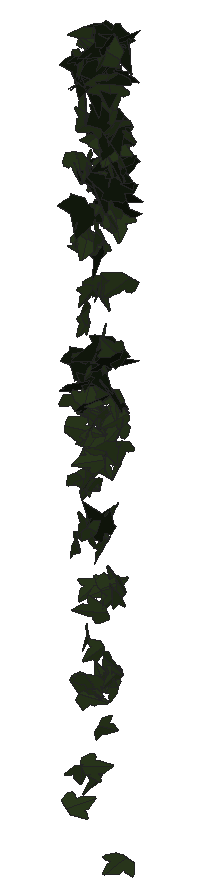
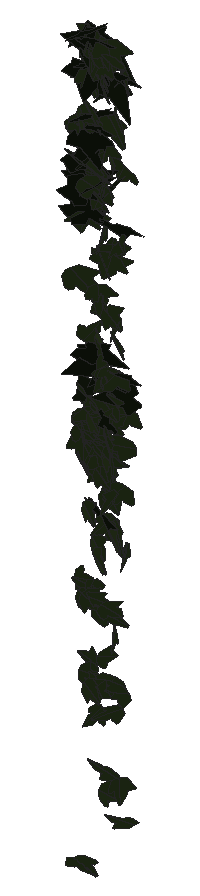
# SketchUp Ruby script. Lengths in inches.
U = 1.inch
M = Sketchup.active_model
def pt(a) = Geom::Point3d.new(a.map { |v| v * U })
def face(e, loops, mat)
  f = e.add_face(loops[0].map { |a| pt(a) })
  loops[1..].each { |l| e.add_face(l.map { |a| pt(a) }).erase! }
  f.material = f.back_material = mat if mat
  f
end
# faces: each face lists its corners as indices into pts; further lists are holes
def faces(e, pts, list, mat = nil) = list.each { |f| face(e, (f[0].is_a?(Array) ? f : [f]).map { |l| l.map { |i| pts[i] } }, mat) }
# xy, xz, yz: faces in a plane at the given z, y or x. An outline is a flat list of corners, or four numbers for a rectangle; further outlines are holes
def ring(l) = l.size == 4 ? [[l[0], l[1]], [l[2], l[1]], [l[2], l[3]], [l[0], l[3]]] : l.each_slice(2).to_a
def flat(e, list, mat, &to3) = list.each { |f| face(e, (f[0].is_a?(Array) ? f : [f]).map { |l| ring(l).map { |u, v| to3.(u, v) } }, mat) }
def xy(e, z, list, mat = nil) = flat(e, list, mat) { |x, y| [x, y, z] }
def xz(e, y, list, mat = nil) = flat(e, list, mat) { |x, z| [x, y, z] }
def yz(e, x, list, mat = nil) = flat(e, list, mat) { |y, z| [x, y, z] }
def lines(e, pts, list) = list.each { |a, b| e.add_line(pt(pts[a]), pt(pts[b])) }
# prism: a flat outline (further loops are holes) pulled along v
def prism(e, loops, v, mat = nil)
  f = face(e, loops, mat); d = Geom::Vector3d.new(v.map { |x| x * U })
  f.pushpull(f.normal.samedirection?(d) ? d.length : -d.length)
end
def box(e, o, s, mat = nil) = prism(e, [[o, [o[0] + s[0], o[1], o[2]], [o[0] + s[0], o[1] + s[1], o[2]], [o[0], o[1] + s[1], o[2]]]], [0, 0, s[2]], mat)
def at(x, y, z, deg = 0) = Geom::Transformation.translation(pt([x, y, z])) * Geom::Transformation.rotation(ORIGIN, Z_AXIS, deg.degrees)
def axes(o, x, y, z) = Geom::Transformation.new([*x, 0, *y, 0, *z, 0, *pt(o).to_a, 1])
def part(name) = M.definitions.add(name)
# library, detail: a bought-in or finely detailed component or shape, given as its bounding box
def library(name, o, s) = part(name).tap { |d| box(d.entities, o, s) }
def detail(e, o, s) = box(e.add_group.entities, o, s)
def put(e, d, t, mat = nil) = e.add_instance(d, t).tap { |i| i.material = mat if mat }
def group(e, t, mat = nil) = e.add_group.tap { |g| g.transformation = t; g.material = mat if mat }.entities
root = M.entities
M.materials.add("1026 AP 7946 SUNNY SIDE UP").color = [254, 231, 186]
M.materials.add("efeu1").color = [18, 25, 13]
M.materials.add("efeu2").color = [43, 57, 29]
c1 = part("ivyleaf_10")
p = [[0,0.5,-0.03],[-0.0625,2.02,-0.43],[-0.19,2.01,-0.46],[-0.54,1.05,-0.29],[-0.52,0.625,-0.18],[-0.83,0.76,-0.28],
  [-1.16,0.64,-0.33],[-1.15,0.33,-0.24],[-0.77,-0.39,0.02],[-0.3,-0.51,0.16],[0.04,-0.48,0.23],[-0.02,2.01,-0.4375],
  [-0.06,2.01,-0.43],[0.04,-0.49,0.23],[0.67,-0.49,0.14],[1.38,0.36,-0.2],[1.375,0.51,-0.24],[0.81,0.65,-0.19],
  [0.62,0.59,-0.15],[0.6,1.09,-0.28],[0.5,1.23,-0.31]]
faces(c1.entities,p,[[0,1,2,3,4,5,6,7,8,9,10],[11,12,0,13,14,15,16,17,18,19,20]],"efeu2")
c2 = part("ivyleaf_9")
p = [[1.54,2.16,1.25],[1.36,2.04,1.19],[-0.21,0.99,0.68],[-0.71,1.11,0.82],[-0.85,0.86,0.67],[-0.8,0.17,0.21],
  [-0.9,-0.01,0.1],[-0.67,-0.16,-0.02],[-0.08,-0.08,-0.05],[-0.03,-0.6,-0.4],[0.65,-0.88,-0.66],[0.83,-0.6,-0.49],
  [1.29,-0.42,-0.43],[1.8125,-0.07,-0.26],[1.21,0.44,0.15]]
faces(c2.entities,p,[[0,1,2,3,4,5,6,7,8,9,10,11,12,13,14]],"efeu1")
put(root,c1,axes([98.51,212.3,259.13],[-0.27937,-0.11894,-0.10126],[0.16168,0.02502,-0.21427],[0.19891,-0.18739,0.03195]),"1026 AP 7946 SUNNY SIDE UP")
put(root,c1,axes([98.56,212.43,263.14],[0.0391,0.17474,-0.14079],[-0.04815,-0.13104,-0.19029],[-0.37047,0.03547,0.00987]),"1026 AP 7946 SUNNY SIDE UP")
put(root,c1,axes([98.64,212.66,261.58],[-0.05241,-0.19052,0.11214],[-0.0155,-0.10979,-0.19972],[0.34552,-0.03382,0.00805]),"1026 AP 7946 SUNNY SIDE UP")
put(root,c1,axes([98.7,212.33,261.15],[-0.02487,0.03429,0.22922],[-0.17054,0.1886,-0.03714],[-0.32536,-0.10148,0.00194]),"1026 AP 7946 SUNNY SIDE UP")
put(root,c1,axes([98.63,212.31,250.48],[-0.13312,-0.18944,-0.0198],[0.02536,0.01265,-0.21346],[0.29817,-0.08566,0.00931]),"1026 AP 7946 SUNNY SIDE UP")
put(root,c1,axes([98.66,212.21,267.14],[0.21762,-0.19818,-0.09251],[-0.05141,0.08493,-0.24763],[0.3375,0.14073,0.02193]),"1026 AP 7946 SUNNY SIDE UP")
put(root,c1,axes([98.61,212.11,255.87],[0.08491,-0.17723,-0.12547],[0.04251,0.12919,-0.18207],[0.33455,0.02856,0.05498]),"1026 AP 7946 SUNNY SIDE UP")
put(root,c1,axes([98.64,212.44,260.89],[0.20499,-0.14401,-0.02204],[-0.03094,0.00911,-0.2009],[0.24458,0.12186,-0.00694]),"1026 AP 7946 SUNNY SIDE UP")
put(root,c2,axes([98.64,212.48,263.58],[-0.31071,-0.12436,-0.07465],[0.13892,-0.00184,-0.23189],[0.19656,-0.19529,0.04589]),"1026 AP 7946 SUNNY SIDE UP")
put(root,c2,axes([98.81,212.31,266.75],[-0.07178,0.25204,-0.03444],[0.00058,-0.03588,-0.27404],[-0.43207,-0.04192,0.00535]),"1026 AP 7946 SUNNY SIDE UP")
put(root,c1,axes([98.47,212.21,249.57],[0.1939,-0.0085,-0.16852],[0.22459,0.10571,0.10591],[0.12594,-0.17543,0.07058]),"1026 AP 7946 SUNNY SIDE UP")
put(root,c1,axes([98.69,212.43,258.09],[0.0331,-0.17595,-0.11475],[-0.0054,0.11064,-0.18171],[0.32656,0.01966,0.00863]),"1026 AP 7946 SUNNY SIDE UP")
put(root,c1,axes([98.75,212.6,254.67],[-0.13776,-0.09753,0.15854],[-0.03053,-0.16535,-0.11989],[0.2856,-0.06472,0.06366]),"1026 AP 7946 SUNNY SIDE UP")
put(root,c2,axes([98.49,212.11,259.4375],[0.25239,0.03969,0.18222],[0.21659,0.12714,-0.14975],[-0.20151,0.18637,0.06728]),"1026 AP 7946 SUNNY SIDE UP")
put(root,c1,axes([98.76,212.52,267.7],[-0.25265,-0.20537,0.01811],[0.0007,-0.02446,-0.27142],[0.35021,-0.14811,0.01361]),"1026 AP 7946 SUNNY SIDE UP")
put(root,c1,axes([98.42,212.33,258.4],[-0.01641,-0.02412,-0.23445],[0.37076,0.02531,-0.01297],[0.04498,-0.21743,0.02139]),"1026 AP 7946 SUNNY SIDE UP")
put(root,c1,axes([98.6,212.31,257.33],[-0.20644,-0.11253,-0.14995],[0.18656,0.08385,-0.17732],[0.22005,-0.17665,0.00967]),"1026 AP 7946 SUNNY SIDE UP")
put(root,c1,axes([98.7,212.56,262.8],[-0.3743,-0.00639,-0.02967],[0.04805,-0.03659,-0.2333],[0.00288,-0.21918,0.03667]),"1026 AP 7946 SUNNY SIDE UP")
put(root,c1,axes([98.91,212.42,258.85],[-0.2398,0.00932,-0.15753],[-0.24756,0.02224,0.15158],[0.03815,0.20285,-0.00651]),"1026 AP 7946 SUNNY SIDE UP")
put(root,c1,axes([98.72,212.42,256.24],[0.1317,-0.18099,0.0391],[0.01121,-0.0396,-0.20543],[0.2909,0.08347,-0.00979]),"1026 AP 7946 SUNNY SIDE UP")
put(root,c1,axes([98.93,212.24,265.76],[-0.29804,0.04713,0.15883],[-0.25334,0.0093,-0.19292],[-0.07154,-0.22927,0.02148]),"1026 AP 7946 SUNNY SIDE UP")
put(root,c1,axes([98.71,212.42,257.18],[-0.01521,0.1355,0.17254],[-0.0448,0.15754,-0.14275],[-0.3523,-0.02588,0.01071]),"1026 AP 7946 SUNNY SIDE UP")
put(root,c2,axes([98.67,212.45,260.06],[-0.25441,-0.13473,-0.09736],[0.13066,0.04743,-0.2145],[0.24116,-0.16783,0.01351]),"1026 AP 7946 SUNNY SIDE UP")
put(root,c1,axes([98.56,212.23,264.79],[0.31903,-0.04945,0.11744],[0.17921,-0.03232,-0.20846],[0.10007,0.21553,-0.00108]),"1026 AP 7946 SUNNY SIDE UP")
put(root,c1,axes([98.92,212.13,256.26],[-0.23981,0.10446,0.18077],[-0.25733,0.06726,-0.18802],[-0.19073,-0.22208,0.02638]),"1026 AP 7946 SUNNY SIDE UP")
put(root,c1,axes([98.81,212.42,262.64],[-0.3139,-0.13165,-0.04887],[-0.07982,-0.0075,0.24533],[-0.20463,0.20488,-0.02072]),"1026 AP 7946 SUNNY SIDE UP")
put(root,c1,axes([98.64,212.48,260.07],[-0.27784,-0.10961,-0.13621],[0.19397,0.04971,-0.213],[0.18681,-0.21463,0.01858]),"1026 AP 7946 SUNNY SIDE UP")
put(root,c1,axes([98.83,212.42,257.21],[-0.11923,-0.19489,0.07201],[-0.02811,-0.06918,-0.21568],[0.32494,-0.07749,0.00777]),"1026 AP 7946 SUNNY SIDE UP")
put(root,c1,axes([98.75,212.36,262.96],[0.24998,0.15657,-0.06162],[-0.04989,-0.05398,-0.2303],[-0.27997,0.14941,-0.01399]),"1026 AP 7946 SUNNY SIDE UP")
put(root,c1,axes([98.75,212.61,258.21],[0.0492,-0.16845,0.14669],[0.07592,-0.13609,-0.17639],[0.33941,0.05486,0.01819]),"1026 AP 7946 SUNNY SIDE UP")
put(root,c2,axes([98.96,212.17,267.46],[-0.18866,0.20878,-0.03742],[0.00466,-0.04111,-0.25315],[-0.3601,-0.10991,0.01633]),"1026 AP 7946 SUNNY SIDE UP")
put(root,c1,axes([98.6,212.42,266.15],[0.16854,-0.13767,0.21387],[0.24806,-0.13848,-0.17866],[0.30445,0.18904,0.02717]),"1026 AP 7946 SUNNY SIDE UP")
put(root,c1,axes([98.83,212.49,258.63],[0.07149,-0.19155,-0.08157],[-0.04031,0.07412,-0.20225],[0.32276,0.05169,-0.00719]),"1026 AP 7946 SUNNY SIDE UP")
put(root,c1,axes([98.95,212.46,259.375],[-0.26546,-0.0683,0.11549],[-0.15441,-0.06207,-0.18262],[0.15391,-0.18008,0.01597]),"1026 AP 7946 SUNNY SIDE UP")
put(root,c1,axes([98.87,212.55,258.04],[-0.2726,-0.1235,0.03485],[-0.03129,-0.03195,-0.21681],[0.21525,-0.16104,0.01263]),"1026 AP 7946 SUNNY SIDE UP")
put(root,c2,axes([98.79,212.36,267.02],[-0.32616,-0.1046,-0.10236],[0.18194,-0.00527,-0.22775],[0.15498,-0.21394,0.05195]),"1026 AP 7946 SUNNY SIDE UP")
put(root,c2,axes([98.65,212.44,264.46],[0.14434,-0.22674,-0.01818],[-0.01554,0.01365,-0.25189],[0.35712,0.09224,-0.00361]),"1026 AP 7946 SUNNY SIDE UP")
put(root,c1,axes([98.68,212.36,252.18],[-0.03252,-0.09944,-0.18967],[0.23523,0.12159,-0.08452],[0.22895,-0.13905,0.05989]),"1026 AP 7946 SUNNY SIDE UP")
put(root,c1,axes([98.79,212.44,257.34],[0.04933,-0.08937,0.20495],[0.08983,-0.19114,-0.09861],[0.33172,0.06505,-0.00378]),"1026 AP 7946 SUNNY SIDE UP")
put(root,c1,axes([98.63,212.25,252.57],[-0.14215,0.00609,-0.19948],[0.29393,-0.05353,-0.09194],[-0.08022,-0.20692,0.01662]),"1026 AP 7946 SUNNY SIDE UP")
put(root,c1,axes([98.79,212.25,259.16],[0.26711,0.08182,-0.04599],[0.05247,0.03555,0.18951],[0.14875,-0.15948,0.01573]),"1026 AP 7946 SUNNY SIDE UP")
put(root,c1,axes([98.88,212.65,257.78],[-0.01609,-0.19014,0.09831],[0.01082,-0.09687,-0.19642],[0.33511,-0.006,0.01106]),"1026 AP 7946 SUNNY SIDE UP")
put(root,c2,axes([98.71,212.31,258.92],[0.14653,0.19149,-0.00182],[-0.02185,0.01039,0.22436],[0.32441,-0.08579,0.01594]),"1026 AP 7946 SUNNY SIDE UP")
put(root,c1,axes([98.82,212.67,261.57],[0.0062,-0.14525,-0.12528],[0.00136,-0.11514,0.15394],[-0.31463,-0.00336,-0.0018]),"1026 AP 7946 SUNNY SIDE UP")
put(root,c1,axes([98.92,212.47,258.3],[0.21092,0.1292,-0.12172],[-0.12844,-0.08725,-0.19305],[-0.26451,0.14539,-0.00332]),"1026 AP 7946 SUNNY SIDE UP")
put(root,c1,axes([98.85,212.51,259.88],[-0.00044,-0.02629,0.21402],[0.09057,-0.19314,-0.02977],[0.33067,0.05287,0.00844]),"1026 AP 7946 SUNNY SIDE UP")
put(root,c1,axes([99.13,212.3125,254.32],[-0.09911,-0.00675,0.21605],[-0.29908,-0.09071,-0.06242],[0.13944,-0.19935,0.01968]),"1026 AP 7946 SUNNY SIDE UP")
put(root,c1,axes([98.9,212.49,250.27],[0.03302,-0.12848,0.16499],[0.02266,-0.1604,-0.13484],[0.32294,0.02439,-0.00741]),"1026 AP 7946 SUNNY SIDE UP")
put(root,c1,axes([99.03,212.33,257.82],[-0.10683,0.00899,0.20822],[-0.1252,-0.19014,-0.01881],[0.30566,-0.07474,0.06507]),"1026 AP 7946 SUNNY SIDE UP")
put(root,c1,axes([98.81,212.34,264.8],[-0.03844,0.04428,-0.23709],[0.06371,-0.21933,-0.05399],[-0.37903,-0.04135,0.01497]),"1026 AP 7946 SUNNY SIDE UP")
put(root,c1,axes([98.85,212.59,267.46],[0.4133,0.0296,-0.00112],[0.0025,-0.02394,-0.26165],[-0.05024,0.24229,-0.02225]),"1026 AP 7946 SUNNY SIDE UP")
put(root,c1,axes([98.95,212.07,253.8],[0.06144,-0.13569,-0.16844],[-0.01402,0.16428,-0.14236],[0.33287,0.03197,0.02509]),"1026 AP 7946 SUNNY SIDE UP")
put(root,c1,axes([98.92,212.65,260.23],[0.01419,0.05061,-0.20662],[-0.05246,-0.19117,-0.05758],[-0.33571,0.03201,0.00027]),"1026 AP 7946 SUNNY SIDE UP")
put(root,c1,axes([98.8125,212.59,266.8],[0.14377,-0.14618,0.19051],[0.17448,-0.14794,-0.18261],[0.35264,0.1328,0.01268]),"1026 AP 7946 SUNNY SIDE UP")
put(root,c1,axes([98.99,212.3,264.31],[-0.1231,0.16229,0.12319],[-0.10423,0.09588,-0.18835],[-0.31906,-0.09394,0.014]),"1026 AP 7946 SUNNY SIDE UP")
put(root,c1,axes([98.97,212.42,258.94],[-0.26949,-0.09574,-0.00046],[0.01282,-0.0141,-0.19793],[0.16202,-0.15813,0.01489]),"1026 AP 7946 SUNNY SIDE UP")
put(root,c1,axes([98.72,212.62,258.68],[0.14584,-0.03881,0.19813],[0.28165,-0.07065,-0.10397],[0.12671,0.2017,0.00307]),"1026 AP 7946 SUNNY SIDE UP")
put(root,c1,axes([98.99,212.55,261.97],[-0.19522,-0.17849,-0.0024],[0.02161,-0.00831,-0.22685],[0.30222,-0.1147,0.01468]),"1026 AP 7946 SUNNY SIDE UP")
put(root,c2,axes([98.78,212.33,259.95],[-0.08489,-0.0751,-0.20496],[0.2101,0.1451,-0.09401],[0.27687,-0.13314,0.0085]),"1026 AP 7946 SUNNY SIDE UP")
put(root,c1,axes([98.93,212.21,252.72],[-0.31487,-0.04415,-0.07122],[0.1122,-0.00511,-0.21034],[0.06296,-0.2117,0.01864]),"1026 AP 7946 SUNNY SIDE UP")
put(root,c1,axes([98.96,212.625,255.76],[0.15168,-0.18378,0.09964],[0.05257,-0.09267,-0.214],[0.32307,0.10136,-0.01196]),"1026 AP 7946 SUNNY SIDE UP")
put(root,c1,axes([98.89,212.6,261.67],[-0.20873,0.08763,-0.10783],[0.10935,-0.08274,-0.1606],[-0.20018,-0.13657,0.02471]),"1026 AP 7946 SUNNY SIDE UP")
put(root,c2,axes([98.82,212.39,266.625],[0.04333,-0.23865,0.0913],[0.01307,-0.08807,-0.25817],[0.43181,0.02662,-0.00135]),"1026 AP 7946 SUNNY SIDE UP")
put(root,c1,axes([99,212.41,253.35],[-0.05101,-0.04646,0.20196],[0.03258,-0.19855,-0.04604],[0.31552,0.01299,0.0374]),"1026 AP 7946 SUNNY SIDE UP")
put(root,c1,axes([98.99,212.5,264.29],[-0.35077,0.08538,-0.0237],[0.02606,-0.02229,-0.24573],[-0.13678,-0.2232,0.01397]),"1026 AP 7946 SUNNY SIDE UP")
put(root,c2,axes([98.95,212.5,262.72],[-0.18407,0.03122,-0.19618],[0.28013,-0.08249,-0.12047],[-0.14672,-0.19667,0.01609]),"1026 AP 7946 SUNNY SIDE UP")
put(root,c1,axes([99,212.5,267.29],[-0.3934,0.08999,-0.04134],[0.04673,-0.03845,-0.26528],[-0.16036,-0.23197,0.02411]),"1026 AP 7946 SUNNY SIDE UP")
put(root,c1,axes([99.15,212.62,254.77],[-0.16653,-0.02914,0.17857],[-0.12282,-0.17366,-0.08019],[0.24787,-0.10563,0.08023]),"1026 AP 7946 SUNNY SIDE UP")
put(root,c1,axes([99.11,212.49,257.97],[-0.11314,-0.17832,0.14224],[-0.06082,-0.1341,-0.19852],[0.35036,-0.08086,0.01147]),"1026 AP 7946 SUNNY SIDE UP")
put(root,c1,axes([99.21,212.61,264.4],[-0.1747,-0.09415,0.19935],[-0.14618,-0.17141,-0.14518],[0.32467,-0.12783,0.0419]),"1026 AP 7946 SUNNY SIDE UP")
put(root,c1,axes([98.9,212.52,259.97],[0.01188,-0.03247,-0.20074],[0.16152,-0.16141,0.03155],[-0.27894,-0.09484,0.00972]),"1026 AP 7946 SUNNY SIDE UP")
put(root,c1,axes([99.09,212.4375,265.28],[-0.39106,-0.06687,-0.01707],[0.03446,-0.01607,-0.25604],[0.11115,-0.2303,0.01932]),"1026 AP 7946 SUNNY SIDE UP")
put(root,c1,axes([99.09,212.35,260.55],[0.14282,-0.13579,0.13688],[-0.09682,0.11684,0.1723],[-0.3036,-0.10113,0.00944]),"1026 AP 7946 SUNNY SIDE UP")
put(root,c1,axes([98.83,212.3,250.59],[0.14585,-0.06022,-0.1841],[0.28577,-0.0232,0.1053],[-0.07717,-0.19969,0.04199]),"1026 AP 7946 SUNNY SIDE UP")
put(root,c1,axes([99.08,212.23,263.22],[0.11176,-0.16866,-0.19047],[0.03383,0.19468,-0.1742],[0.39094,0.03137,0.06953]),"1026 AP 7946 SUNNY SIDE UP")
put(root,c2,axes([99.26,212.54,260.47],[0.00297,-0.01479,-0.25364],[-0.11877,-0.23433,0.01254],[-0.36907,0.07529,-0.00607]),"1026 AP 7946 SUNNY SIDE UP")
put(root,c1,axes([99.02,212.39,257.8],[-0.20222,-0.14229,-0.09098],[0.15478,0.02853,-0.19177],[0.23302,-0.14244,0.04843]),"1026 AP 7946 SUNNY SIDE UP")
put(root,c1,axes([99.18,212.41,252.55],[0.29749,0.01746,0.10047],[-0.15501,0.01435,0.19465],[0.01398,-0.21232,0.02016]),"1026 AP 7946 SUNNY SIDE UP")
put(root,c1,axes([99.35,212.52,264.85],[-0.28601,0.07589,-0.16491],[-0.22965,0.07649,0.19856],[0.18198,0.2158,-0.00862]),"1026 AP 7946 SUNNY SIDE UP")
put(root,c1,axes([99.16,212.55,258.93],[0.0244,-0.20982,0.06757],[0.01133,-0.06642,-0.21712],[0.34604,0.01697,0.00234]),"1026 AP 7946 SUNNY SIDE UP")
put(root,c1,axes([99.13,212.47,264.1],[0.30419,-0.18857,0.02078],[0.00339,-0.02815,-0.27782],[0.29837,0.19257,-0.01803]),"1026 AP 7946 SUNNY SIDE UP")
put(root,c1,axes([98.9,212.65,258.17],[0.05188,-0.04894,-0.23021],[0.2716,-0.14227,0.05761],[-0.23518,-0.1751,0.01575]),"1026 AP 7946 SUNNY SIDE UP")
put(root,c1,axes([99.17,212.66,252.7],[0.00421,-0.19365,0.09972],[0.00482,-0.09786,-0.20008],[0.34116,0.00377,0.0016]),"1026 AP 7946 SUNNY SIDE UP")
put(root,c1,axes([99.25,212.49,263.65],[-0.33224,0.00236,-0.05382],[-0.08442,0.02268,0.20861],[0.01343,0.2008,-0.02009]),"1026 AP 7946 SUNNY SIDE UP")
put(root,c2,axes([99.23,212.53,265.48],[0.17339,0.14884,-0.14041],[-0.10257,-0.11944,-0.19431],[-0.32305,0.11781,-0.01366]),"1026 AP 7946 SUNNY SIDE UP")
put(root,c2,axes([99.39,212.09,256.4],[-0.05623,0.09418,0.24728],[-0.1681,0.21451,-0.10209],[-0.36809,-0.11235,0.00885]),"1026 AP 7946 SUNNY SIDE UP")
put(root,c1,axes([99.1875,212.39,255.95],[0.01516,-0.19879,0.05062],[-0.00178,-0.05038,-0.2053],[0.32242,0.00907,-0.00351]),"1026 AP 7946 SUNNY SIDE UP")
put(root,c2,axes([99.07,212.52,264.36],[-0.04317,-0.23907,0.01891],[-0.00146,-0.01973,-0.24802],[0.37718,-0.02744,0.0012]),"1026 AP 7946 SUNNY SIDE UP")
put(root,c1,axes([99.09,212.0625,256.36],[-0.12191,-0.12486,-0.16671],[0.15397,0.12836,-0.15028],[0.2811,-0.12446,0.01002]),"1026 AP 7946 SUNNY SIDE UP")
put(root,c1,axes([99.19,212.6875,254.8],[-0.05059,-0.16572,0.15327],[0.02261,-0.15248,-0.17159],[0.35044,-0.01409,0.0332]),"1026 AP 7946 SUNNY SIDE UP")
put(root,c2,axes([99.28,212.63,267.72],[-0.37175,-0.09723,0.01009],[-0.00117,-0.02468,-0.25575],[0.16604,-0.21786,0.02078]),"1026 AP 7946 SUNNY SIDE UP")
put(root,c1,axes([98.94,212.48,266.82],[0.14659,-0.09669,0.20939],[0.30651,-0.08873,-0.1327],[0.21131,0.19579,0.04723]),"1026 AP 7946 SUNNY SIDE UP")
put(root,c1,axes([99.125,212.46,267.72],[-0.14475,0.19883,-0.07155],[0.0347,-0.06673,-0.23242],[-0.35582,-0.0874,0.00644]),"1026 AP 7946 SUNNY SIDE UP")
put(root,c1,axes([99.35,212.63,258.81],[0.04839,0.08916,0.22234],[-0.17094,-0.18662,0.09452],[0.32414,-0.11173,0.01666]),"1026 AP 7946 SUNNY SIDE UP")
put(root,c1,axes([99.55,212.2,267.56],[0.07075,0.07181,0.27262],[-0.44743,0.0041,0.04517],[0.01263,-0.25708,0.07301]),"1026 AP 7946 SUNNY SIDE UP")
put(root,c1,axes([99.42,212.32,263.47],[-0.19613,0.08259,-0.15324],[-0.18402,0.09568,0.15298],[0.21384,0.15809,-0.0089]),"1026 AP 7946 SUNNY SIDE UP")
put(root,c1,axes([99.27,212.34,267.43],[-0.00084,-0.19379,-0.15786],[0.01382,0.14484,-0.20534],[0.41055,-0.00527,0.00659]),"1026 AP 7946 SUNNY SIDE UP")
put(root,c1,axes([99.3,212.46,266.08],[0.25064,-0.19225,-0.05334],[-0.06549,0.02996,-0.25877],[0.32965,0.15213,-0.01085]),"1026 AP 7946 SUNNY SIDE UP")
put(root,c1,axes([99.3,212.32,266.87],[-0.20472,-0.22447,-0.00255],[0.02293,-0.00788,-0.27239],[0.38035,-0.12034,0.01505]),"1026 AP 7946 SUNNY SIDE UP")
put(root,c1,axes([99.13,212.47,264.63],[0.26061,-0.10514,0.1217],[0.1574,-0.06819,-0.20013],[0.21266,0.17932,-0.00102]),"1026 AP 7946 SUNNY SIDE UP")
put(root,c1,axes([99.1875,212.41,257.9],[0.01978,-0.07689,-0.17308],[0.04168,-0.15878,0.08104],[-0.29948,-0.02718,-0.00015]),"1026 AP 7946 SUNNY SIDE UP")
put(root,c1,axes([99.26,212.48,264.75],[0.3648,-0.06025,-0.03795],[-0.04196,0.04111,-0.24438],[0.10251,0.23123,0.03504]),"1026 AP 7946 SUNNY SIDE UP")
put(root,c1,axes([99.28,212.48,266.84],[-0.20561,-0.17786,-0.04612],[0.0578,0.02603,-0.22958],[0.30432,-0.12512,0.01244]),"1026 AP 7946 SUNNY SIDE UP")
put(root,c2,axes([99.4,212.41,267.69],[-0.01814,-0.02384,-0.24178],[-0.01211,-0.22563,0.02274],[-0.38478,0.00822,0.01068]),"1026 AP 7946 SUNNY SIDE UP")
put(root,c2,axes([99.57,212.5,264.84],[-0.22791,0.17836,0.08616],[-0.16261,0.02215,-0.23],[-0.2878,-0.15376,0.06173]),"1026 AP 7946 SUNNY SIDE UP")
put(root,c2,axes([99.15,212.33,260.12],[0.19177,0.12467,0.19431],[0.2139,0.12971,-0.17885],[-0.2828,0.18265,-0.00351]),"1026 AP 7946 SUNNY SIDE UP")
put(root,c2,axes([99.29,212.47,266.95],[0.27351,0.12665,-0.08236],[-0.0845,-0.06335,-0.21946],[-0.23849,0.16769,-0.01669]),"1026 AP 7946 SUNNY SIDE UP")
put(root,c1,axes([99.45,212.31,252.69],[0.1287,-0.1055,-0.18228],[-0.19127,0.1281,-0.13638],[0.26041,0.14623,-0.01009]),"1026 AP 7946 SUNNY SIDE UP")
put(root,c2,axes([99.13,212.63,265.08],[0.10328,-0.23495,0.07659],[0.01956,-0.07506,-0.25163],[0.38764,0.06638,-0.00771]),"1026 AP 7946 SUNNY SIDE UP")
put(root,c1,axes([99.38,212.55,254.74],[-0.06566,-0.15869,0.12767],[-0.03589,-0.12294,-0.1696],[0.31544,-0.04702,0.00728]),"1026 AP 7946 SUNNY SIDE UP")
put(root,c2,axes([99.34,212.54,265.64],[-0.32122,-0.1331,-0.05703],[0.09117,0.01289,-0.24658],[0.22448,-0.19569,0.01854]),"1026 AP 7946 SUNNY SIDE UP")
put(root,c2,axes([99.24,212.4,267.04],[-0.17957,-0.21721,-0.06582],[0.07597,0.04319,-0.2571],[0.3743,-0.11298,0.02061]),"1026 AP 7946 SUNNY SIDE UP")
put(root,c2,axes([99.46,212.65,264.97],[0.00581,0.03068,-0.22619],[-0.05785,-0.20892,-0.03592],[-0.35845,0.03421,0.00213]),"1026 AP 7946 SUNNY SIDE UP")
put(root,c1,axes([99.35,212.49,256.74],[0.04266,-0.19718,0.04041],[0.00153,-0.04058,-0.20523],[0.31646,0.02677,-0.00446]),"1026 AP 7946 SUNNY SIDE UP")
put(root,c1,axes([99.39,212.63,258.63],[-0.16,-0.12796,0.14919],[-0.01055,-0.16196,-0.15247],[0.30454,-0.07284,0.0731]),"1026 AP 7946 SUNNY SIDE UP")
put(root,c1,axes([99.31,212.41,265.33],[0.35199,0.11081,-0.04219],[-0.04906,-0.03241,-0.25165],[-0.19438,0.20883,-0.01287]),"1026 AP 7946 SUNNY SIDE UP")
put(root,c1,axes([99.28,212.62,267.65],[-0.11009,0.15606,-0.14731],[0.05327,-0.13728,-0.18179],[-0.35147,-0.06969,0.01859]),"1026 AP 7946 SUNNY SIDE UP")
put(root,c2,axes([99.22,212.48,265.94],[-0.05004,-0.26045,-0.06169],[0.04666,0.055,-0.26901],[0.4171,-0.0374,0.02269]),"1026 AP 7946 SUNNY SIDE UP")
put(root,c2,axes([99.22,212.6,263.625],[0.36445,0.05152,0.05962],[-0.09964,0.0101,0.23524],[0.08027,-0.2214,0.02134]),"1026 AP 7946 SUNNY SIDE UP")
put(root,c2,axes([99.4375,212.44,267.39],[-0.22001,0.11891,-0.1482],[0.14513,-0.11257,-0.18869],[-0.27595,-0.15401,0.01892]),"1026 AP 7946 SUNNY SIDE UP")
put(root,c2,axes([99.62,212.41,264.3],[-0.06496,0.0317,0.24073],[-0.3823,-0.03122,-0.03682],[0.04379,-0.22554,0.03566]),"1026 AP 7946 SUNNY SIDE UP")
put(root,c1,axes([99.45,212.37,254.85],[-0.27113,0.09803,0.06226],[-0.09769,0.01125,-0.20323],[-0.15193,-0.18218,0.01957]),"1026 AP 7946 SUNNY SIDE UP")
put(root,c1,axes([99.46,212.59,258.9],[-0.08876,-0.06904,0.19994],[-0.0495,-0.19638,-0.08238],[0.3207,-0.04942,0.04262]),"1026 AP 7946 SUNNY SIDE UP")
put(root,c1,axes([99.57,212.42,254.97],[-0.14733,0.06868,-0.19372],[-0.20375,0.13801,0.11901],[0.24069,0.15887,-0.01783]),"1026 AP 7946 SUNNY SIDE UP")
put(root,c1,axes([99.2,212.41,254.89],[0.16012,0.04224,-0.16986],[0.22812,0.08637,0.11097],[0.16171,-0.16366,0.01165]),"1026 AP 7946 SUNNY SIDE UP")
put(root,c1,axes([99.5,212.29,260.59],[-0.14678,-0.11322,-0.13078],[-0.15384,-0.08153,0.15026],[-0.23503,0.12407,-0.01668]),"1026 AP 7946 SUNNY SIDE UP")
put(root,c1,axes([99.42,212.49,252.9],[-0.02392,-0.08654,0.18857],[0.03389,-0.1837,-0.08847],[0.31725,0.0131,0.02367]),"1026 AP 7946 SUNNY SIDE UP")
put(root,c1,axes([99.64,212.51,265.45],[-0.21414,0.01047,-0.17514],[-0.27329,0.03185,0.13542],[0.05361,0.20422,-0.00921]),"1026 AP 7946 SUNNY SIDE UP")
put(root,c1,axes([99.36,212.07,251.82],[-0.06269,-0.1078,-0.18966],[0.12261,0.16629,-0.11714],[0.31135,-0.08719,0.00794]),"1026 AP 7946 SUNNY SIDE UP")
put(root,c1,axes([99.58,212.55,262.13],[-0.22454,-0.14903,0.15779],[-0.14943,-0.12185,-0.21295],[0.30205,-0.17107,0.01195]),"1026 AP 7946 SUNNY SIDE UP")
put(root,c1,axes([99.46,212.53,265.76],[-0.19921,-0.19053,0.01184],[0.01009,-0.01953,-0.23928],[0.32409,-0.1165,0.01473]),"1026 AP 7946 SUNNY SIDE UP")
put(root,c1,axes([99.45,212.46,258.27],[-0.25921,-0.17441,-0.00869],[0.02601,-0.00541,-0.24674],[0.27326,-0.16493,0.01524]),"1026 AP 7946 SUNNY SIDE UP")
put(root,c1,axes([99.47,212.54,258.74],[0.12526,-0.18036,-0.08359],[-0.03962,0.07639,-0.20254],[0.30778,0.08324,0.00794]),"1026 AP 7946 SUNNY SIDE UP")
put(root,c1,axes([99.5,212.55,248.5],[0.26648,0.04057,-0.11421],[-0.16048,-0.04792,-0.1787],[-0.09397,0.19689,-0.01869]),"1026 AP 7946 SUNNY SIDE UP")
put(root,c1,axes([99.4,212.58,257.86],[0.18828,-0.15279,0.07771],[0.05552,-0.06903,-0.19988],[0.26274,0.12408,-0.01345]),"1026 AP 7946 SUNNY SIDE UP")
put(root,c1,axes([99.37,212.51,263.59],[0.15545,0.23092,-0.00664],[0.00924,-0.01094,-0.25865],[-0.36319,0.09856,-0.00942]),"1026 AP 7946 SUNNY SIDE UP")
put(root,c1,axes([99.3,212.53,259.36],[0.27508,-0.07215,0.12455],[0.16206,-0.06668,-0.19437],[0.15161,0.20217,-0.0182]),"1026 AP 7946 SUNNY SIDE UP")
put(root,c1,axes([99.21,212.41,253.15],[-0.0056,-0.00999,0.2107],[0.31096,-0.05343,0.00055],[0.08383,0.19751,0.01205]),"1026 AP 7946 SUNNY SIDE UP")
put(root,c2,axes([99.28,212.51,267.88],[0.04283,-0.26313,-0.08502],[0.02918,0.083,-0.27074],[0.43194,0.02048,0.02672]),"1026 AP 7946 SUNNY SIDE UP")
put(root,c1,axes([99.48,212.2,266.75],[-0.3085,-0.14653,-0.02859],[0.05389,-0.00001,-0.24902],[0.24645,-0.18342,0.01866]),"1026 AP 7946 SUNNY SIDE UP")
put(root,c2,axes([99.26,212.58,264.08],[0.38285,0.03507,-0.00349],[-0.0003,0.02519,0.24324],[0.05987,-0.22415,0.02354]),"1026 AP 7946 SUNNY SIDE UP")
put(root,c2,axes([99.28,212.53,259.45],[-0.00162,-0.16708,0.18213],[0.10616,-0.17099,-0.16619],[0.36859,0.04851,0.04867]),"1026 AP 7946 SUNNY SIDE UP")
put(root,c2,axes([99.35,212.32,267.5],[0.03409,0.01156,0.26138],[0.29021,0.1742,-0.02147],[-0.29617,0.17202,0.00905]),"1026 AP 7946 SUNNY SIDE UP")
put(root,c1,axes([99.51,212.4,265.84],[0.02059,-0.24625,0.03497],[0.00184,-0.03586,-0.26444],[0.42242,0.01216,-0.00055]),"1026 AP 7946 SUNNY SIDE UP")
